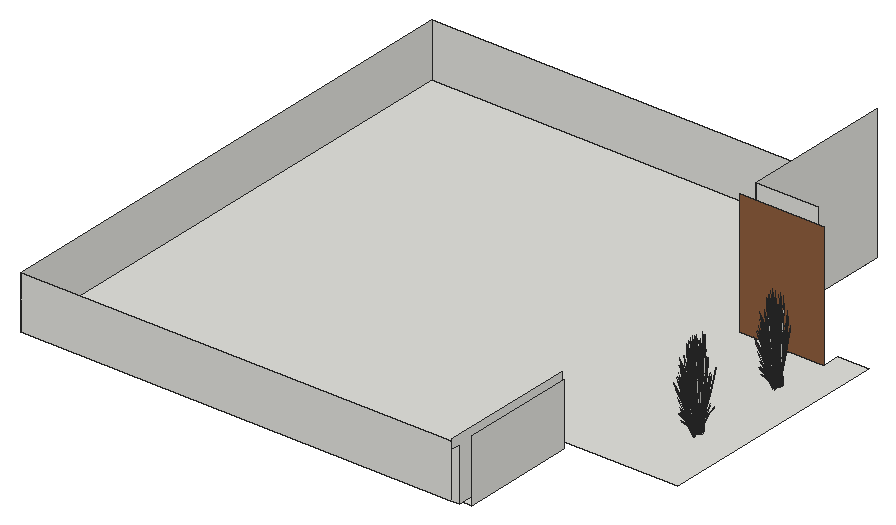
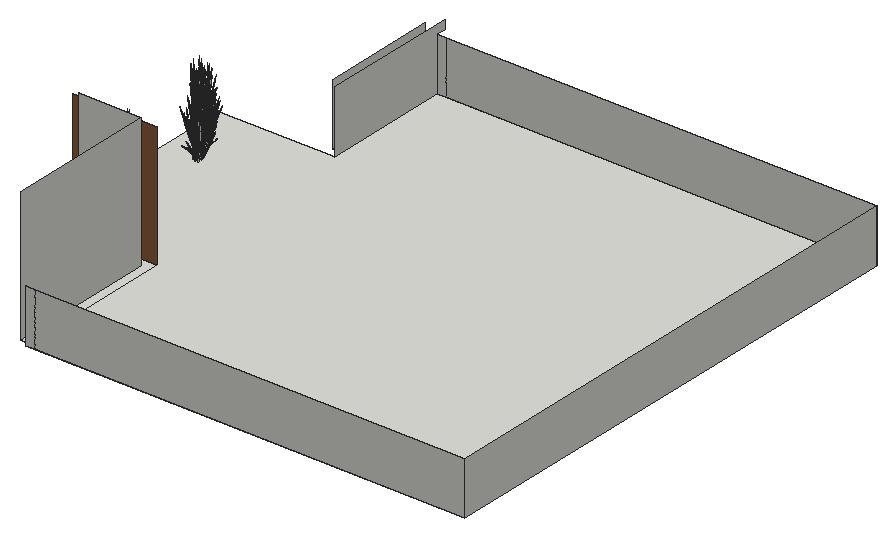
# SketchUp Ruby script. Lengths in inches.
U = 1.inch
M = Sketchup.active_model
def pt(a) = Geom::Point3d.new(a.map { |v| v * U })
def face(e, loops, mat)
  f = e.add_face(loops[0].map { |a| pt(a) })
  loops[1..].each { |l| e.add_face(l.map { |a| pt(a) }).erase! }
  f.material = f.back_material = mat if mat
  f
end
# faces: each face lists its corners as indices into pts; further lists are holes
def faces(e, pts, list, mat = nil) = list.each { |f| face(e, (f[0].is_a?(Array) ? f : [f]).map { |l| l.map { |i| pts[i] } }, mat) }
# xy, xz, yz: faces in a plane at the given z, y or x. An outline is a flat list of corners, or four numbers for a rectangle; further outlines are holes
def ring(l) = l.size == 4 ? [[l[0], l[1]], [l[2], l[1]], [l[2], l[3]], [l[0], l[3]]] : l.each_slice(2).to_a
def flat(e, list, mat, &to3) = list.each { |f| face(e, (f[0].is_a?(Array) ? f : [f]).map { |l| ring(l).map { |u, v| to3.(u, v) } }, mat) }
def xy(e, z, list, mat = nil) = flat(e, list, mat) { |x, y| [x, y, z] }
def xz(e, y, list, mat = nil) = flat(e, list, mat) { |x, z| [x, y, z] }
def yz(e, x, list, mat = nil) = flat(e, list, mat) { |y, z| [x, y, z] }
def lines(e, pts, list) = list.each { |a, b| e.add_line(pt(pts[a]), pt(pts[b])) }
# prism: a flat outline (further loops are holes) pulled along v
def prism(e, loops, v, mat = nil)
  f = face(e, loops, mat); d = Geom::Vector3d.new(v.map { |x| x * U })
  f.pushpull(f.normal.samedirection?(d) ? d.length : -d.length)
end
def box(e, o, s, mat = nil) = prism(e, [[o, [o[0] + s[0], o[1], o[2]], [o[0] + s[0], o[1] + s[1], o[2]], [o[0], o[1] + s[1], o[2]]]], [0, 0, s[2]], mat)
def at(x, y, z, deg = 0) = Geom::Transformation.translation(pt([x, y, z])) * Geom::Transformation.rotation(ORIGIN, Z_AXIS, deg.degrees)
def axes(o, x, y, z) = Geom::Transformation.new([*x, 0, *y, 0, *z, 0, *pt(o).to_a, 1])
def part(name) = M.definitions.add(name)
# library, detail: a bought-in or finely detailed component or shape, given as its bounding box
def library(name, o, s) = part(name).tap { |d| box(d.entities, o, s) }
def detail(e, o, s) = box(e.add_group.entities, o, s)
def put(e, d, t, mat = nil) = e.add_instance(d, t).tap { |i| i.material = mat if mat }
def group(e, t, mat = nil) = e.add_group.tap { |g| g.transformation = t; g.material = mat if mat }.entities
root = M.entities
M.materials.add("LightPink_Translucent").color = [144, 107, 117]
M.materials["LightPink_Translucent"].alpha = 0.75
M.materials.add("Wood_Veneer_15_1K").color = [142, 95, 62]
c1 = part("blade")
p = [[2.15,0.21,22],[0,0.17,0],[0.09,0.45,0],[2.18,0.31,22],[2.29,0.31,22],[0.38,0.45,0],
  [2.48,0.24,33],[2.49,0.24,33],[2.48,0.22,33]]
faces(c1.entities,p,[[0,1,2,3],[4,5,2,3],[6,3,4,7],[8,0,3,6]])
c2 = part("seeds")
p = [[0.3,-0.1,1.38],[-0.01,-0.03,1.59],[-0.01,-0.03,0.03],[0.14,-0.07,-0.07],[0.29,-0.03,3],[0.15,0.01,3.11]]
faces(c2.entities,p,[[0,1,2,3],[1,0,4,5]],"LightPink_Translucent")
c3 = part("blade with seeds")
put(c3.entities,c1,at(0,0,0))
put(c3.entities,c2,axes([2.4,0.25,30.99],[1.5799,-0.05474,1.17369],[-0.12525,1.92788,0.29478],[-0.07173,-0.02425,1.56792]))
xy(root,402,[[6,6,303,6,303,93,381,93,381,255,360,255,360,243,303,243,303,354,6,354],[303,9,309,87],[303,243,303,351,309,351,309,249,351,249,351,243]])
xz(root,6,[[6,402,297,438],[297,402,303,438]])
xz(root,243,[[303,402,360,486]],"Wood_Veneer_15_1K")
xz(root,249,[[309,402,351,492]])
xz(root,354,[[6,402,297,438],[297,402,303,438]])
yz(root,6,[[6,402,354,438]])
yz(root,303,[[6,402,6,438,0,438,0,444,93,444,93,402]])
yz(root,309,[[9,402,87,444],[249,402,351,492]])
p = [[297,351,402],[297,354,402]]
lines(root,p,[[0,1]])
put(root,c3,axes([354.2,140.67,405.64],[0.20312,-0.01367,1.61094],[-0.13474,0.59258,0.13026],[-0.28946,-0.03665,0.68866]))
put(root,c3,axes([354.28,141.71,405.64],[0.16991,-0.12769,1.61094],[0.14304,0.59005,0.13026],[-0.26674,0.13336,0.68866]))
put(root,c3,axes([353.76,142.71,404.44],[0.17018,0.04956,1.34422],[0.10969,0.50618,-0.28909],[-0.23117,0.09475,0.57472]))
put(root,c3,axes([355.26,141.09,405.14],[0.13919,-0.08733,1.6644],[0.048,0.60974,0.13026],[-0.3015,0.08091,0.59487]))
put(root,c3,axes([353.76,141.5,406.43],[-0.07997,0.07838,1.64448],[0.0068,0.57266,-0.26007],[-0.1833,0.07447,0.13189]))
put(root,c3,axes([354.81,140.11,406.68],[-0.48951,-0.01454,-0.66783],[0.03288,-0.61207,0.08059],[-0.20738,-0.06459,0.9447]))
put(root,c3,axes([354.41,140.26,404.44],[0.09561,0.16807,1.34422],[-0.22031,0.45686,-0.28909],[-0.22622,-0.1092,0.57472]))
put(root,c3,axes([354.02,141.17,406.25],[-0.40696,-0.16841,-0.33289],[0.1187,-0.49132,0.42977],[-0.16385,0.04505,0.82232]))
put(root,c3,axes([354.58,139.71,405.64],[0.1819,0.10401,1.61094],[-0.37643,0.43634,0.13026],[-0.23461,-0.19684,0.68866]))
put(root,c3,axes([352.875,142.08,406.43],[0.06249,0.01619,1.6674],[0.19333,0.53339,-0.15755],[-0.12793,0.14,0.29507]))
put(root,c3,axes([354.3,141.42,406.4],[-0.13266,0.54912,-0.48033],[-0.45484,-0.18822,-0.37205],[-0.18313,0.05035,0.91906]))
put(root,c3,axes([354.64,140.24,406.4],[-0.35558,0.39989,-0.48033],[-0.31141,-0.42243,-0.37205],[-0.18066,-0.06084,0.91906]))
put(root,c3,axes([354.07,141.39,403.4],[0.01242,0.09514,1.65762],[-0.25036,0.49684,-0.25323],[-0.17783,-0.02504,0.28235]))
put(root,c3,axes([354.14,139.12,406.43],[0.0363,0.06025,1.6674],[-0.17501,0.54156,-0.15755],[-0.17724,0.00392,0.29507]))
put(root,c3,axes([353.4,143.77,404.6],[0.20408,-0.2736,1.07969],[0.08053,0.43313,0.79328],[-0.14748,0.07756,0.23781]))
put(root,c3,axes([354.55,138.76,406.43],[-0.10536,-0.00426,1.64448],[-0.33544,0.42612,-0.26007],[-0.17898,-0.08707,0.13189]))
put(root,c3,axes([356.14,205.96,405.64],[0.20312,-0.01367,1.61094],[-0.13474,0.59258,0.13026],[-0.28946,-0.03665,0.68866]))
put(root,c3,axes([354.12,141.11,406.45],[0.13835,-0.55043,0.45122],[0.45484,0.18822,0.37205],[-0.17887,0.03308,0.9337]))
put(root,c3,axes([354.28,140.96,406.73],[0.24639,0.54664,-0.11431],[-0.43729,0.26863,-0.63445],[-0.18428,0.07212,0.96403]))
put(root,c3,axes([354.83,139.82,406.73],[-0.02622,0.61393,-0.11431],[-0.49645,-0.01678,-0.63445],[-0.1912,-0.04265,0.96403]))
put(root,c3,axes([354.51,139.86,406.25],[-0.27863,-0.37797,-0.33289],[0.31815,-0.35779,0.42977],[-0.16164,-0.05444,0.82232]))
put(root,c3,axes([354.08,140.97,406.45],[-0.17985,-0.41162,0.06044],[0.32797,-0.20147,0.47584],[-0.14457,0.03975,0.72558]))
put(root,c3,axes([354.91,142.11,405.64],[0.12231,-0.18549,1.61094],[0.30882,0.50067,0.13026],[-0.21182,0.22801,0.68866]))
put(root,c3,axes([354.17,142.59,406.25],[-0.42626,0.08628,-0.33289],[-0.11256,-0.4932,0.42977],[-0.12215,0.13247,0.82232]))
put(root,c3,axes([353.9375,144.05,403.4],[0.06569,0.06031,1.65762],[0.11138,0.55882,-0.25323],[-0.14558,0.11917,0.28235]))
put(root,c3,axes([353.84,140.77,404.6],[0.31263,-0.0432,1.07969],[-0.19831,0.38061,0.79328],[-0.15449,-0.0571,0.23781]))
put(root,c3,axes([354.23,142.48,406.45],[-0.12145,-0.5556,0.45122],[0.4764,-0.09643,0.37205],[-0.14041,0.13067,0.9337]))
put(root,c3,axes([356.23,207,405.64],[0.16991,-0.12769,1.61094],[0.14304,0.59005,0.13026],[-0.26674,0.13336,0.68866]))
put(root,c3,axes([354.47,139.72,406.79],[0.4044,-0.44551,0.50537],[0.34877,0.47312,0.4167],[-0.18973,-0.08218,1.04574]))
put(root,c3,axes([354.13,142.38,406.45],[-0.33617,-0.25389,0.06044],[0.19572,-0.36154,0.47584],[-0.10778,0.11689,0.72558]))
put(root,c3,axes([355.7,208.01,404.44],[0.17018,0.04956,1.34422],[0.10969,0.50618,-0.28909],[-0.23117,0.09475,0.57472]))
put(root,c3,axes([354.8125,142.5625,405.64],[0.09118,-0.2075,1.61094],[0.3825,0.42941,0.13026],[-0.17255,0.26763,0.68866]))
put(root,c3,axes([357.2,206.38,405.14],[0.13919,-0.08733,1.6644],[0.048,0.60974,0.13026],[-0.3015,0.08091,0.59487]))
put(root,c3,axes([354.45,141.12,406.75],[0.40696,0.16841,0.33289],[-0.1187,0.49132,-0.42977],[-0.16385,0.04505,0.82232]))
put(root,c3,axes([354.52,142.65,406.4],[0.1258,0.55122,-0.48033],[-0.4764,0.09643,-0.37205],[-0.13652,0.14806,0.91906]))
put(root,c3,axes([354.66,139.72,406.45],[0.02466,-0.45905,0.06044],[0.37234,0.01259,0.47584],[-0.14263,-0.04803,0.72558]))
put(root,c3,axes([353.78,143.64,406.43],[-0.01217,0.11946,1.64448],[0.34544,0.41559,-0.26007],[-0.09043,0.19653,0.13189]))
put(root,c3,axes([355.71,142.25,403.9375],[-0.50939,-0.09897,-0.58612],[0.10749,-0.61051,-0.15383],[-0.15202,-0.07398,1.29375]))
put(root,c3,axes([355.8,138.92,407.1],[-0.32682,0.57873,-0.12802],[-0.47329,-0.33342,-0.71058],[-0.16452,-0.16351,1.07972]))
put(root,c3,axes([355.71,206.79,406.43],[-0.07997,0.07838,1.64448],[0.0068,0.57266,-0.26007],[-0.1833,0.07447,0.13189]))
put(root,c3,axes([356.75,205.41,406.68],[-0.48951,-0.01454,-0.66783],[0.03288,-0.61207,0.08059],[-0.20738,-0.06459,0.9447]))
put(root,c3,axes([354.91,140.06,406.75],[0.27863,0.37797,0.33289],[-0.31815,0.35779,-0.42977],[-0.16164,-0.05444,0.82232]))
put(root,c3,axes([356.36,205.56,404.44],[0.09561,0.16807,1.34422],[-0.22031,0.45686,-0.28909],[-0.22622,-0.1092,0.57472]))
put(root,c3,axes([355.66,139.39,406.68],[-0.41756,-0.29179,-0.66783],[0.29675,-0.51132,0.08059],[-0.15128,-0.17422,0.9447]))
put(root,c3,axes([355.46,139.41,406.4],[-0.48321,0.1435,-0.48033],[-0.08453,-0.54345,-0.37205],[-0.12979,-0.15574,0.91906]))
put(root,c3,axes([355.97,206.47,406.25],[-0.40696,-0.16841,-0.33289],[0.1187,-0.49132,0.42977],[-0.16385,0.04505,0.82232]))
put(root,c3,axes([356.53,205.01,405.64],[0.1819,0.10401,1.61094],[-0.37643,0.43634,0.13026],[-0.23461,-0.19684,0.68866]))
put(root,c3,axes([355.04,143.41,403.9],[-0.4583,-0.30184,-0.46672],[0.27394,-0.54125,0],[-0.10438,-0.06875,1.48054]))
put(root,c3,axes([354.84,138.91,403.4],[-0.04743,0.07953,1.65762],[-0.47936,0.17146,-0.25323],[-0.1158,-0.15598,0.28235]))
put(root,c3,axes([354.3,142.25,406.73],[0.45297,0.33287,-0.11431],[-0.26096,0.48206,-0.63445],[-0.12798,0.16757,0.96403]))
put(root,c3,axes([354.82,207.37,406.43],[0.06249,0.01619,1.6674],[0.19333,0.53339,-0.15755],[-0.12793,0.14,0.29507]))
put(root,c3,axes([356.24,206.72,406.4],[-0.13266,0.54912,-0.48033],[-0.45484,-0.18822,-0.37205],[-0.18313,0.05035,0.91906]))
put(root,c3,axes([355.32,143.77,404.23],[-0.30616,0.60492,0],[-0.51222,-0.33735,-0.48511],[-0.11666,-0.07683,1.53889]))
put(root,c3,axes([356.59,205.53,406.4],[-0.35558,0.39989,-0.48033],[-0.31141,-0.42243,-0.37205],[-0.18066,-0.06084,0.91906]))
put(root,c3,axes([356.02,206.68,403.4],[0.01242,0.09514,1.65762],[-0.25036,0.49684,-0.25323],[-0.17783,-0.02504,0.28235]))
put(root,c3,axes([353.55,143.7,407.31],[0.43212,0.16114,-0.06098],[-0.13292,0.49597,-0.27651],[-0.07068,0.0753,0.91203]))
put(root,c3,axes([356.09,204.41,406.43],[0.0363,0.06025,1.6674],[-0.17501,0.54156,-0.15755],[-0.17724,0.00392,0.29507]))
put(root,c3,axes([354.52,142.3,406.75],[0.42626,-0.08628,0.33289],[0.11256,0.4932,-0.42977],[-0.12215,0.13247,0.82232]))
put(root,c3,axes([355.34,209.07,404.6],[0.20408,-0.2736,1.07969],[0.08053,0.43313,0.79328],[-0.14748,0.07756,0.23781]))
put(root,c3,axes([354.76,144.65,404.44],[0.15453,-0.09523,1.34422],[0.38153,0.28715,-0.28909],[-0.11356,0.24846,0.57472]))
put(root,c3,axes([356.49,204.05,406.43],[-0.10536,-0.00426,1.64448],[-0.33544,0.42612,-0.26007],[-0.17898,-0.08707,0.13189]))
put(root,c3,axes([354.54,139.22,404],[-0.14126,0.49294,-0.03659],[-0.43477,-0.15163,-0.1659],[-0.06601,-0.08063,0.54722]))
put(root,c3,axes([356.06,206.41,406.45],[0.13835,-0.55043,0.45122],[0.45484,0.18822,0.37205],[-0.17887,0.03308,0.9337]))
put(root,c3,axes([356.22,206.25,406.73],[0.24639,0.54664,-0.11431],[-0.43729,0.26863,-0.63445],[-0.18428,0.07212,0.96403]))
put(root,c3,axes([355.67,137.55,406.43],[-0.00914,0.07236,1.6674],[-0.45057,0.26261,-0.15755],[-0.13259,-0.13424,0.29507]))
put(root,c3,axes([356.78,205.11,406.73],[-0.02622,0.61393,-0.11431],[-0.49645,-0.01678,-0.63445],[-0.1912,-0.04265,0.96403]))
put(root,c3,axes([356.46,205.16,406.25],[-0.27863,-0.37797,-0.33289],[0.31815,-0.35779,0.42977],[-0.16164,-0.05444,0.82232]))
put(root,c3,axes([356.03,206.26,406.45],[-0.17985,-0.41162,0.06044],[0.32797,-0.20147,0.47584],[-0.14457,0.03975,0.72558]))
put(root,c3,axes([355.19,138.6,404.44],[-0.02965,0.19748,1.34422],[-0.43351,0.16532,-0.28909],[-0.10133,-0.25525,0.57472]))
put(root,c3,axes([356.85,207.4,405.64],[0.12231,-0.18549,1.61094],[0.30882,0.50067,0.13026],[-0.21182,0.22801,0.68866]))
put(root,c3,axes([356.11,207.88,406.25],[-0.42626,0.08628,-0.33289],[-0.11256,-0.4932,0.42977],[-0.12215,0.13247,0.82232]))
put(root,c3,axes([355.33,139.11,405.64],[0.11194,0.19382,1.61094],[-0.51725,0.16318,0.13026],[-0.1169,-0.30428,0.68866]))
put(root,c3,axes([356.29,142.34,404.51],[-0.49442,0.40079,-0.2735],[-0.32878,-0.56631,-0.47002],[-0.12199,-0.05751,1.50125]))
put(root,c3,axes([354.92,143.61,406.45],[-0.3487,-0.41189,0.45122],[0.37031,-0.35523,0.37205],[-0.06432,0.19325,0.9337]))
put(root,c3,axes([355.88,209.35,403.4],[0.06569,0.06031,1.65762],[0.11138,0.55882,-0.25323],[-0.14558,0.11917,0.28235]))
put(root,c3,axes([355.51,139.01,406.25],[-0.07563,-0.48625,-0.33289],[0.43235,-0.1284,0.42977],[-0.11613,-0.13934,0.82232]))
put(root,c3,axes([355.79,206.0625,404.6],[0.31263,-0.0432,1.07969],[-0.19831,0.38061,0.79328],[-0.15449,-0.0571,0.23781]))
put(root,c3,axes([354.31,141.47,404.23],[-0.61233,0,0],[0,-0.67471,-0.48511],[0,-0.15367,1.53889]))
put(root,c3,axes([355.17,143.18,403.91],[-0.11503,-0.52602,-0.29119],[0.45686,-0.14937,0.29119],[-0.0921,-0.06066,1.30635]))
put(root,c3,axes([354.79,143.57,406.45],[-0.40242,-0.02813,0.06044],[0.01103,-0.42474,0.47584],[-0.04211,0.1627,0.72558]))
put(root,c3,axes([354.92,143.73,406.25],[-0.33133,0.31784,-0.33289],[-0.31365,-0.36292,0.42977],[-0.04772,0.1844,0.82232]))
put(root,c3,axes([356.17,207.78,406.45],[-0.12145,-0.5556,0.45122],[0.4764,-0.09643,0.37205],[-0.14041,0.13067,0.9337]))
put(root,c3,axes([356.42,205.01,406.79],[0.4044,-0.44551,0.50537],[0.34877,0.47312,0.4167],[-0.18973,-0.08218,1.04574]))
put(root,c3,axes([356.62,142.78,403.9375],[-0.32983,0.45375,-0.58612],[-0.40974,-0.41145,-0.15383],[-0.13217,0.11319,1.29375]))
put(root,c3,axes([356.08,207.67,406.45],[-0.33617,-0.25389,0.06044],[0.19572,-0.36154,0.47584],[-0.10778,0.11689,0.72558]))
put(root,c3,axes([355.77,139.4,406.75],[0.07563,0.48625,0.33289],[-0.43235,0.1284,-0.42977],[-0.11613,-0.13934,0.82232]))
put(root,c3,axes([353.74,144.86,406.43],[0.05555,-0.03645,1.6674],[0.45917,0.24243,-0.15755],[-0.01079,0.20185,0.29507]))
put(root,c3,axes([354.78,141.29,404.19],[-0.45549,0.50754,0.28911],[-0.45577,-0.5022,-0.34302],[-0.01591,-0.14413,1.54992]))
put(root,c3,axes([356.66,142.69,405.125],[0.42317,0.24343,1.42185],[-0.41456,0.52443,0.56227],[-0.18569,-0.31082,1.19198]))
put(root,c3,axes([356.76,207.86,405.64],[0.09118,-0.2075,1.61094],[0.3825,0.42941,0.13026],[-0.17255,0.26763,0.68866]))
put(root,c3,axes([355.04,138.28,404.6],[0.25544,0.21011,1.07969],[-0.37201,0.1263,0.79328],[-0.0796,-0.16148,0.23781]))
put(root,c3,axes([356.84,142.53,404.32],[-0.47817,-0.48589,-0.23681],[0.40236,-0.54561,0.51822],[-0.12876,0.05684,1.58123]))
put(root,c3,axes([355.97,142.06,404.08],[-0.29417,-0.5067,-0.42055],[0.44558,-0.35681,0.2024],[-0.0952,-0.0627,1.35025]))
put(root,c3,axes([355.14,143.4,407.02],[-0.01274,0.55841,-0.74129],[-0.53656,-0.0375,0.08946],[-0.05662,0.23657,1.04862]))
put(root,c3,axes([356.39,206.41,406.75],[0.40696,0.16841,0.33289],[-0.1187,0.49132,-0.42977],[-0.16385,0.04505,0.82232]))
put(root,c3,axes([355.13,144.97,404.6],[-0.01267,-0.35895,1.07969],[0.31667,0.25602,0.79328],[-0.06228,0.17109,0.23781]))
put(root,c3,axes([355.58,138.83,406.79],[0.5455,-0.15516,0.50537],[0.09467,0.60867,0.4167],[-0.12829,-0.17939,1.04574]))
put(root,c3,axes([356.47,207.94,406.4],[0.1258,0.55122,-0.48033],[-0.4764,0.09643,-0.37205],[-0.13652,0.14806,0.91906]))
put(root,c3,axes([356.6,142.42,404.08],[-0.53176,0.03727,-0.42055],[-0.04809,-0.6186,0.2024],[-0.0952,0.0627,1.35025]))
put(root,c3,axes([356.6,205.01,406.45],[0.02466,-0.45905,0.06044],[0.37234,0.01259,0.47584],[-0.14263,-0.04803,0.72558]))
put(root,c3,axes([355.72,208.93,406.43],[-0.01217,0.11946,1.64448],[0.34544,0.41559,-0.26007],[-0.09043,0.19653,0.13189]))
put(root,c3,axes([357.65,207.55,403.9375],[-0.50939,-0.09897,-0.58612],[0.10749,-0.61051,-0.15383],[-0.15202,-0.07398,1.29375]))
put(root,c3,axes([357.75,204.22,407.1],[-0.32682,0.57873,-0.12802],[-0.47329,-0.33342,-0.71058],[-0.16452,-0.16351,1.07972]))
put(root,c3,axes([355.7,138.96,406.45],[0.22256,-0.38349,0.06044],[0.31694,0.22327,0.47584],[-0.10247,-0.12295,0.72558]))
put(root,c3,axes([356.85,205.35,406.75],[0.27863,0.37797,0.33289],[-0.31815,0.35779,-0.42977],[-0.16164,-0.05444,0.82232]))
put(root,c3,axes([355.58,143.46,404.33],[0.4583,0.30184,0.46672],[-0.27394,0.54125,0],[-0.10438,-0.06875,1.48054]))
put(root,c3,axes([354.96,144.18,405.16],[0.01076,-0.31164,1.45085],[0.48391,0.16461,0.20049],[-0.04193,0.33214,0.68509]))
put(root,c3,axes([357.6,204.6875,406.68],[-0.41756,-0.29179,-0.66783],[0.29675,-0.51132,0.08059],[-0.15128,-0.17422,0.9447]))
put(root,c3,axes([357.41,204.7,406.4],[-0.48321,0.1435,-0.48033],[-0.08453,-0.54345,-0.37205],[-0.12979,-0.15574,0.91906]))
put(root,c3,axes([356.02,142.35,404.29],[0.12979,-0.71533,-0.22023],[0.6154,0.12469,0.48194],[-0.10753,-0.09879,1.47054]))
put(root,c3,axes([356.24,142.52,404.46],[-0.09447,0.53876,0.13611],[-0.46155,-0.09352,-0.38866],[-0.084,-0.05532,1.1914]))
put(root,c3,axes([356.99,208.7,403.9],[-0.4583,-0.30184,-0.46672],[0.27394,-0.54125,0],[-0.10438,-0.06875,1.48054]))
put(root,c3,axes([356.78,204.21,403.4],[-0.04743,0.07953,1.65762],[-0.47936,0.17146,-0.25323],[-0.1158,-0.15598,0.28235]))
put(root,c3,axes([356.24,207.55,406.73],[0.45297,0.33287,-0.11431],[-0.26096,0.48206,-0.63445],[-0.12798,0.16757,0.96403]))
put(root,c3,axes([356.1875,137.82,406.43],[-0.0749,-0.08464,1.64448],[-0.49984,0.05366,-0.26007],[-0.07977,-0.20245,0.13189]))
put(root,c3,axes([357.16,144.02,403.9],[-0.4583,0.30184,-0.46672],[-0.27394,-0.54125,0],[-0.10438,0.06875,1.48054]))
put(root,c3,axes([354.45,141.01,403.9],[0,-0.60368,-0.46672],[0.54787,0,0],[0,-0.13749,1.48054]))
put(root,c3,axes([354.68,141.57,404.33],[0,0.60368,0.46672],[-0.54787,0,0],[0,-0.13749,1.48054]))
put(root,c3,axes([357.1875,143.86,404.0625],[-0.30235,-0.60704,-0.04834],[0.51222,-0.33735,0.48511],[-0.12622,0.0578,1.53813]))
put(root,c3,axes([357.26,209.07,404.23],[-0.30616,0.60492,0],[-0.51222,-0.33735,-0.48511],[-0.11666,-0.07683,1.53889]))
put(root,c3,axes([355.25,143.58,406.7],[0.35055,0.40562,-0.53317],[-0.37031,0.35523,-0.41298],[-0.05334,0.20609,1.02016]))
put(root,c3,axes([357.05,143.78,403.91],[-0.45686,-0.14937,-0.29119],[0.11503,-0.52602,0.29119],[-0.0921,0.06066,1.30635]))
put(root,c3,axes([355.09,143.28,406.75],[0.33133,-0.31784,0.33289],[0.31365,0.36292,-0.42977],[-0.04772,0.1844,0.82232]))
put(root,c3,axes([355.49,208.99,407.31],[0.43212,0.16114,-0.06098],[-0.13292,0.49597,-0.27651],[-0.07068,0.0753,0.91203]))
put(root,c3,axes([355.88,141.71,404.51],[-0.55148,-0.28805,-0.2735],[0.26554,-0.60796,-0.47002],[-0.01733,-0.14927,1.50125]))
put(root,c3,axes([357.3125,141.53,404.67],[-0.01338,-0.56839,1.32796],[0.60542,0.14734,0.56227],[-0.14319,0.31102,1.25349]))
put(root,c3,axes([356.46,207.59,406.75],[0.42626,-0.08628,0.33289],[0.11256,0.4932,-0.42977],[-0.12215,0.13247,0.82232]))
put(root,c3,axes([356.71,209.94,404.44],[0.15453,-0.09523,1.34422],[0.38153,0.28715,-0.28909],[-0.11356,0.24846,0.57472]))
put(root,c3,axes([354.88,143.37,407.07],[0.53819,0.02991,-0.12688],[-0.01471,0.56632,-0.70424],[-0.03738,0.21811,1.07008]))
put(root,c3,axes([356.49,204.51,404],[-0.14126,0.49294,-0.03659],[-0.43477,-0.15163,-0.1659],[-0.06601,-0.08063,0.54722]))
put(root,c3,axes([354.87,144.19,404.65],[0.44486,-0.1069,0.06117],[0.10227,0.43069,-0.81126],[-0.0282,0.21802,0.72719]))
put(root,c3,axes([356.97,142.26,404.51],[0.05706,0.68884,-0.2735],[-0.59432,0.04165,-0.47002],[-0.10465,0.09176,1.50125]))
put(root,c3,axes([355.63,141.1,403.97],[-0.2011,-0.61905,-0.65645],[0.5793,-0.22295,-0.17229],[-0.02223,-0.20963,1.449]))
put(root,c3,axes([356.95,139.13,406.73],[-0.47919,0.28106,-0.11431],[-0.23549,-0.49884,-0.63445],[-0.06322,-0.21021,0.96403]))
put(root,c3,axes([356.54,139.16,406.4],[-0.48137,-0.15133,-0.48033],[0.165,-0.51886,-0.37205],[-0.04414,-0.2089,0.91906]))
put(root,c3,axes([357.62,202.84,406.43],[-0.00914,0.07236,1.6674],[-0.45057,0.26261,-0.15755],[-0.13259,-0.13424,0.29507]))
put(root,c3,axes([355.65,143,405.64],[-0.01199,-0.2317,1.61094],[0.51947,0.15371,0.13026],[-0.03213,0.3302,0.68866]))
put(root,c3,axes([357.14,203.89,404.44],[-0.02965,0.19748,1.34422],[-0.43351,0.16532,-0.28909],[-0.10133,-0.25525,0.57472]))
put(root,c3,axes([357.28,204.4,405.64],[0.11194,0.19382,1.61094],[-0.51725,0.16318,0.13026],[-0.1169,-0.30428,0.68866]))
put(root,c3,axes([358.23,207.64,404.51],[-0.49442,0.40079,-0.2735],[-0.32878,-0.56631,-0.47002],[-0.12199,-0.05751,1.50125]))
put(root,c3,axes([354.68,141.02,403.91],[0.34183,-0.37665,-0.29119],[0.34183,0.37665,0.29119],[0,-0.12132,1.30635]))
put(root,c3,axes([356.87,208.9,406.45],[-0.3487,-0.41189,0.45122],[0.37031,-0.35523,0.37205],[-0.06432,0.19325,0.9337]))
put(root,c3,axes([356.22,138.59,404],[-0.3384,0.34633,-0.03659],[-0.31006,-0.3793,-0.1659],[-0.02183,-0.10747,0.54722]))
put(root,c3,axes([356.09,142,404.22],[0.61893,0.12719,0.43009],[-0.12596,0.71835,0.16877],[-0.09045,-0.06936,1.49325]))
put(root,c3,axes([357.46,204.3,406.25],[-0.07563,-0.48625,-0.33289],[0.43235,-0.1284,0.42977],[-0.11613,-0.13934,0.82232]))
put(root,c3,axes([356.25,206.76,404.23],[-0.61233,0,0],[0,-0.67471,-0.48511],[0,-0.15367,1.53889]))
put(root,c3,axes([357.11,208.48,403.91],[-0.11503,-0.52602,-0.29119],[0.45686,-0.14937,0.29119],[-0.0921,-0.06066,1.30635]))
put(root,c3,axes([356.74,208.86,406.45],[-0.40242,-0.02813,0.06044],[0.01103,-0.42474,0.47584],[-0.04211,0.1627,0.72558]))
put(root,c3,axes([356.86,209.03,406.25],[-0.33133,0.31784,-0.33289],[-0.31365,-0.36292,0.42977],[-0.04772,0.1844,0.82232]))
put(root,c3,axes([355.93,141.875,404.56],[-0.23759,0.54397,0.42055],[-0.49367,-0.26179,-0.2024],[0,-0.12539,1.35025]))
put(root,c3,axes([356.71,139.25,406.68],[-0.23372,-0.49086,-0.66783],[0.48111,-0.27356,0.08059],[-0.05465,-0.23717,0.9447]))
put(root,c3,axes([358.56,208.07,403.9375],[-0.32983,0.45375,-0.58612],[-0.40974,-0.41145,-0.15383],[-0.13217,0.11319,1.29375]))
put(root,c3,axes([357.71,204.7,406.75],[0.07563,0.48625,0.33289],[-0.43235,0.1284,-0.42977],[-0.11613,-0.13934,0.82232]))
put(root,c3,axes([355.68,210.16,406.43],[0.05555,-0.03645,1.6674],[0.45917,0.24243,-0.15755],[-0.01079,0.20185,0.29507]))
put(root,c3,axes([356.73,206.58,404.19],[-0.45549,0.50754,0.28911],[-0.45577,-0.5022,-0.34302],[-0.01591,-0.14413,1.54992]))
put(root,c3,axes([355.76,143.15,404.33],[0.52621,-0.16023,0.16584],[0.12993,0.59629,0.32981],[-0.04693,-0.08688,1.50782]))
put(root,c3,axes([358.6,207.99,405.125],[0.42317,0.24343,1.42185],[-0.41456,0.52443,0.56227],[-0.18569,-0.31082,1.19198]))
put(root,c3,axes([356.43,143.25,404.0625],[-0.49367,-0.27103,0],[0.23759,-0.56315,0],[0,0,1.52945]))
put(root,c3,axes([356.8,139.33,406.75],[-0.14763,0.46424,0.33289],[-0.4307,-0.1354,-0.42977],[-0.03949,-0.18691,0.82232]))
put(root,c3,axes([357.57,143.93,404.23],[0.30616,0.60492,0],[-0.51222,0.33735,-0.48511],[-0.11666,0.07683,1.53889]))
put(root,c3,axes([356.99,203.57,404.6],[0.25544,0.21011,1.07969],[-0.37201,0.1263,0.79328],[-0.0796,-0.16148,0.23781]))
put(root,c3,axes([358.79,207.82,404.32],[-0.47817,-0.48589,-0.23681],[0.40236,-0.54561,0.51822],[-0.12876,0.05684,1.58123]))
put(root,c3,axes([357.92,207.35,404.08],[-0.29417,-0.5067,-0.42055],[0.44558,-0.35681,0.2024],[-0.0952,-0.0627,1.35025]))
put(root,c3,axes([356.02,144.1875,406.76],[-0.48252,-0.15782,0.50086],[0.165,-0.51886,0.41298],[0.029,0.20404,1.03641]))
put(root,c3,axes([357.09,208.6875,407.02],[-0.01274,0.55841,-0.74129],[-0.53656,-0.0375,0.08946],[-0.05662,0.23657,1.04862]))
put(root,c3,axes([355.89,144.23,406.45],[-0.36083,0.20517,0.06044],[-0.17661,-0.37413,0.47584],[0.03485,0.16492,0.72558]))
put(root,c3,axes([357.08,210.26,404.6],[-0.01267,-0.35895,1.07969],[0.31667,0.25602,0.79328],[-0.06228,0.17109,0.23781]))
put(root,c3,axes([357.52,204.125,406.79],[0.5455,-0.15516,0.50537],[0.09467,0.60867,0.4167],[-0.12829,-0.17939,1.04574]))
put(root,c3,axes([357.32,143.19,404.33],[0.14146,-0.59996,0.16584],[0.51766,0.16978,0.32981],[-0.08942,0.00292,1.50782]))
put(root,c3,axes([357.08,142.39,404.46],[0.36178,0.36271,0.13611],[-0.30177,0.40921,-0.38866],[-0.084,0.05532,1.1914]))
put(root,c3,axes([358.54,207.72,404.08],[-0.53176,0.03727,-0.42055],[-0.04809,-0.6186,0.2024],[-0.0952,0.0627,1.35025]))
put(root,c3,axes([356.95,141.94,404.16],[-0.45549,-0.5196,-0.05763],[0.45577,-0.51991,0],[-0.01591,-0.01814,1.65037]))
put(root,c3,axes([357.07,142.125,404.56],[0.53176,-0.03727,0.42055],[0.04809,0.6186,-0.2024],[-0.0952,0.0627,1.35025]))
put(root,c3,axes([357.65,204.26,406.45],[0.22256,-0.38349,0.06044],[0.31694,0.22327,0.47584],[-0.10247,-0.12295,0.72558]))
put(root,c3,axes([357.2,143.55,404.19],[0.61306,0.19622,0.28911],[-0.15337,0.70136,-0.34302],[-0.10147,0.08778,1.54992]))
put(root,c3,axes([356.31,138.17,403.4],[-0.08214,0.02175,1.65762],[-0.45422,-0.24483,-0.25323],[0.00762,-0.20421,0.28235]))
put(root,c3,axes([357.53,208.75,404.33],[0.4583,0.30184,0.46672],[-0.27394,0.54125,0],[-0.10438,-0.06875,1.48054]))
put(root,c3,axes([356.91,209.48,405.16],[0.01076,-0.31164,1.45085],[0.48391,0.16461,0.20049],[-0.04193,0.33214,0.68509]))
put(root,c3,axes([357.47,143.51,404.33],[0.4583,-0.30184,0.46672],[0.27394,0.54125,0],[-0.10438,0.06875,1.48054]))
put(root,c3,axes([357.96,207.64,404.29],[0.12979,-0.71533,-0.22023],[0.6154,0.12469,0.48194],[-0.10753,-0.09879,1.47054]))
put(root,c3,axes([356.76,138.84,406.25],[0.14763,-0.46424,-0.33289],[0.4307,0.1354,0.42977],[-0.03949,-0.18691,0.82232]))
put(root,c3,axes([356.03,141.34,404.22],[0.2129,0.67504,0.43009],[-0.60833,0.23474,0.16877],[0.00743,-0.12404,1.49325]))
put(root,c3,axes([355.9375,141.26,404.08],[0.23759,-0.54397,-0.42055],[0.49367,0.26179,0.2024],[0,-0.12539,1.35025]))
put(root,c3,axes([356.55,143.01,404.07],[-0.15978,-0.52046,0],[0.45625,-0.18226,0],[0,0,1.45109]))
put(root,c3,axes([355.96,144.11,403.4],[0.07925,-0.03285,1.65762],[0.47671,0.18081,-0.25323],[0.01394,0.20378,0.28235]))
put(root,c3,axes([358.18,207.8125,404.46],[-0.09447,0.53876,0.13611],[-0.46155,-0.09352,-0.38866],[-0.084,-0.05532,1.1914]))
put(root,c3,axes([358.13,203.12,406.43],[-0.0749,-0.08464,1.64448],[-0.49984,0.05366,-0.26007],[-0.07977,-0.20245,0.13189]))
put(root,c3,axes([356.07,144.29,406.25],[-0.14763,0.46424,-0.33289],[-0.4307,-0.1354,0.42977],[0.03949,0.18691,0.82232]))
put(root,c3,axes([359.1,209.3125,403.9],[-0.4583,0.30184,-0.46672],[-0.27394,-0.54125,0],[-0.10438,0.06875,1.48054]))
put(root,c3,axes([356.39,206.3,403.9],[0,-0.60368,-0.46672],[0.54787,0,0],[0,-0.13749,1.48054]))
put(root,c3,axes([356.625,206.86,404.33],[0,0.60368,0.46672],[-0.54787,0,0],[0,-0.13749,1.48054]))
put(root,c3,axes([359.13,209.15,404.0625],[-0.30235,-0.60704,-0.04834],[0.51222,-0.33735,0.48511],[-0.12622,0.0578,1.53813]))
put(root,c3,axes([357.19,208.875,406.7],[0.35055,0.40562,-0.53317],[-0.37031,0.35523,-0.41298],[-0.05334,0.20609,1.02016]))
put(root,c3,axes([359,209.07,403.91],[-0.45686,-0.14937,-0.29119],[0.11503,-0.52602,0.29119],[-0.0921,0.06066,1.30635]))
put(root,c3,axes([357.04,208.57,406.75],[0.33133,-0.31784,0.33289],[0.31365,0.36292,-0.42977],[-0.04772,0.1844,0.82232]))
put(root,c3,axes([357.19,141.99,404.08],[-0.23759,0.54397,-0.42055],[-0.49367,-0.26179,0.2024],[0,0.12539,1.35025]))
put(root,c3,axes([357.82,207,404.51],[-0.55148,-0.28805,-0.2735],[0.26554,-0.60796,-0.47002],[-0.01733,-0.14927,1.50125]))
put(root,c3,axes([359.26,206.82,404.67],[-0.01338,-0.56839,1.32796],[0.60542,0.14734,0.56227],[-0.14319,0.31102,1.25349]))
put(root,c3,axes([356.9375,138.91,406.45],[0.36083,-0.20517,0.06044],[0.17661,0.37413,0.47584],[-0.03485,-0.16492,0.72558]))
put(root,c3,axes([355.76,145.12,406.43],[0.06207,0.09721,1.64448],[0.50093,0.03819,-0.26007],[0.05037,0.21439,0.13189]))
put(root,c3,axes([358.13,141.65,404.33],[-0.38474,-0.43973,0.16584],[0.38772,-0.42651,0.32981],[-0.04249,0.0898,1.50782]))
put(root,c3,axes([356.83,208.66,407.07],[0.53819,0.02991,-0.12688],[-0.01471,0.56632,-0.70424],[-0.03738,0.21811,1.07008]))
put(root,c3,axes([356.8,141.4,404.07],[0,-0.69851,0],[0.61233,0,0],[0,0,1.68689]))
put(root,c3,axes([356.81,138.94,406.45],[0.48252,0.15782,0.45122],[-0.165,0.51886,0.37205],[-0.029,-0.20404,0.9337]))
put(root,c3,axes([356.8125,209.48,404.65],[0.44486,-0.1069,0.06117],[0.10227,0.43069,-0.81126],[-0.0282,0.21802,0.72719]))
put(root,c3,axes([356.23,141.53,404.29],[0.55175,0.29259,0.22621],[-0.26554,0.60796,0.47002],[0,-0.14015,1.5091]))
put(root,c3,axes([357.11,141.68,404.15],[0,0.69816,-0.05299],[-0.61233,0,0],[0,0.02194,1.68606]))
put(root,c3,axes([358.92,207.55,404.51],[0.05706,0.68884,-0.2735],[-0.59432,0.04165,-0.47002],[-0.10465,0.09176,1.50125]))
put(root,c3,axes([356.05,141.12,404.56],[-0.53176,0.03727,0.42055],[-0.04809,-0.6186,-0.2024],[0.0952,-0.0627,1.35025]))
put(root,c3,axes([357.58,206.39,403.97],[-0.2011,-0.61905,-0.65645],[0.5793,-0.22295,-0.17229],[-0.02223,-0.20963,1.449]))
put(root,c3,axes([358.89,204.42,406.73],[-0.47919,0.28106,-0.11431],[-0.23549,-0.49884,-0.63445],[-0.06322,-0.21021,0.96403]))
put(root,c3,axes([358.48,204.45,406.4],[-0.48137,-0.15133,-0.48033],[0.165,-0.51886,-0.37205],[-0.04414,-0.2089,0.91906]))
put(root,c3,axes([356.02,143.8,406.75],[0.14763,-0.46424,0.33289],[0.4307,0.1354,-0.42977],[0.03949,0.18691,0.82232]))
put(root,c3,axes([357.59,208.29,405.64],[-0.01199,-0.2317,1.61094],[0.51947,0.15371,0.13026],[-0.03213,0.3302,0.68866]))
put(root,c3,axes([355.81,140.06,404.33],[-0.14146,0.59996,0.16584],[-0.51766,-0.16978,0.32981],[0.08942,-0.00292,1.50782]))
put(root,c3,axes([356.82,143.03,404.15],[0.2129,0.69353,-0.05652],[-0.60833,0.24302,0],[0.00743,0.02422,1.61843]))
put(root,c3,axes([356.625,206.32,403.91],[0.34183,-0.37665,-0.29119],[0.34183,0.37665,0.29119],[0,-0.12132,1.30635]))
put(root,c3,axes([358.17,203.88,404],[-0.3384,0.34633,-0.03659],[-0.31006,-0.3793,-0.1659],[-0.02183,-0.10747,0.54722]))
put(root,c3,axes([358.03,207.3,404.22],[0.61893,0.12719,0.43009],[-0.12596,0.71835,0.16877],[-0.09045,-0.06936,1.49325]))
put(root,c3,axes([355.55,139.32,404.23],[-0.30616,-0.60492,0],[0.51222,-0.33735,-0.48511],[0.11666,-0.07683,1.53889]))
put(root,c3,axes([356.11,143.875,406.68],[0.23372,0.49086,-0.66783],[-0.48111,0.27356,0.08059],[0.05465,0.23717,0.9447]))
put(root,c3,axes([358.57,142.12,404.07],[-0.61202,-0.00483,-0.04678],[0,-0.67471,0.46946],[-0.01923,0.15359,1.48851]))
put(root,c3,axes([357.87,207.17,404.56],[-0.23759,0.54397,0.42055],[-0.49367,-0.26179,-0.2024],[0,-0.12539,1.35025]))
put(root,c3,axes([358.66,204.55,406.68],[-0.23372,-0.49086,-0.66783],[0.48111,-0.27356,0.08059],[-0.05465,-0.23717,0.9447]))
